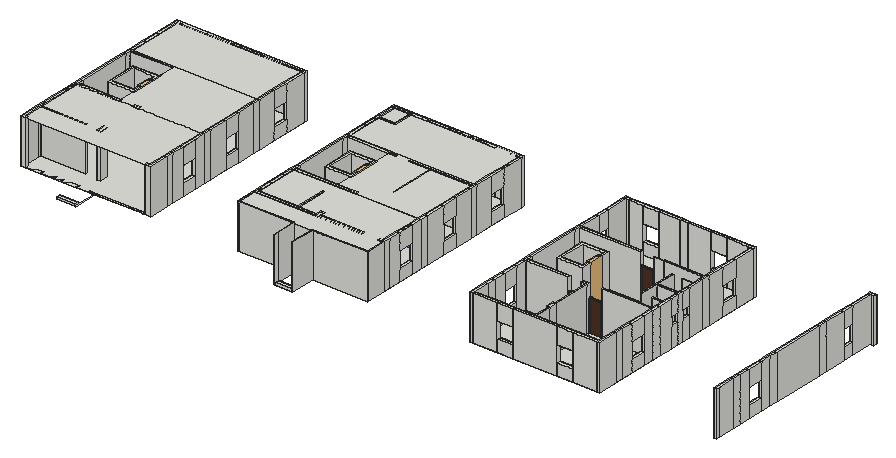
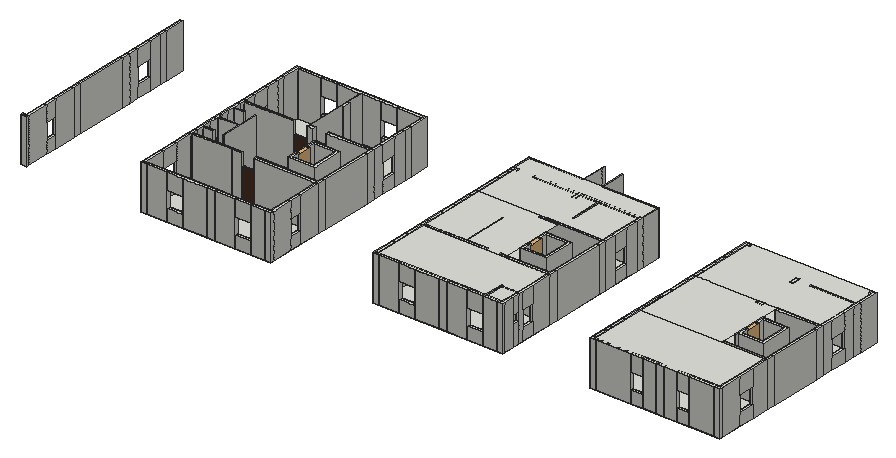
# SketchUp Ruby script. Lengths in inches.
U = 1.inch
M = Sketchup.active_model
def pt(a) = Geom::Point3d.new(a.map { |v| v * U })
def face(e, loops, mat)
  f = e.add_face(loops[0].map { |a| pt(a) })
  loops[1..].each { |l| e.add_face(l.map { |a| pt(a) }).erase! }
  f.material = f.back_material = mat if mat
  f
end
# faces: each face lists its corners as indices into pts; further lists are holes
def faces(e, pts, list, mat = nil) = list.each { |f| face(e, (f[0].is_a?(Array) ? f : [f]).map { |l| l.map { |i| pts[i] } }, mat) }
# xy, xz, yz: faces in a plane at the given z, y or x. An outline is a flat list of corners, or four numbers for a rectangle; further outlines are holes
def ring(l) = l.size == 4 ? [[l[0], l[1]], [l[2], l[1]], [l[2], l[3]], [l[0], l[3]]] : l.each_slice(2).to_a
def flat(e, list, mat, &to3) = list.each { |f| face(e, (f[0].is_a?(Array) ? f : [f]).map { |l| ring(l).map { |u, v| to3.(u, v) } }, mat) }
def xy(e, z, list, mat = nil) = flat(e, list, mat) { |x, y| [x, y, z] }
def xz(e, y, list, mat = nil) = flat(e, list, mat) { |x, z| [x, y, z] }
def yz(e, x, list, mat = nil) = flat(e, list, mat) { |y, z| [x, y, z] }
def lines(e, pts, list) = list.each { |a, b| e.add_line(pt(pts[a]), pt(pts[b])) }
# prism: a flat outline (further loops are holes) pulled along v
def prism(e, loops, v, mat = nil)
  f = face(e, loops, mat); d = Geom::Vector3d.new(v.map { |x| x * U })
  f.pushpull(f.normal.samedirection?(d) ? d.length : -d.length)
end
def box(e, o, s, mat = nil) = prism(e, [[o, [o[0] + s[0], o[1], o[2]], [o[0] + s[0], o[1] + s[1], o[2]], [o[0], o[1] + s[1], o[2]]]], [0, 0, s[2]], mat)
def at(x, y, z, deg = 0) = Geom::Transformation.translation(pt([x, y, z])) * Geom::Transformation.rotation(ORIGIN, Z_AXIS, deg.degrees)
def axes(o, x, y, z) = Geom::Transformation.new([*x, 0, *y, 0, *z, 0, *pt(o).to_a, 1])
def part(name) = M.definitions.add(name)
# library, detail: a bought-in or finely detailed component or shape, given as its bounding box
def library(name, o, s) = part(name).tap { |d| box(d.entities, o, s) }
def detail(e, o, s) = box(e.add_group.entities, o, s)
def put(e, d, t, mat = nil) = e.add_instance(d, t).tap { |i| i.material = mat if mat }
def group(e, t, mat = nil) = e.add_group.tap { |g| g.transformation = t; g.material = mat if mat }.entities
root = M.entities
M.materials.add("Polis06_194").color = [79, 50, 36]
M.materials.add("[Metal Aluminum Anodized]").color = [202, 209, 219]
M.materials.add("[Translucent Glass Blue]").color = [100, 149, 237]
M.materials["[Translucent Glass Blue]"].alpha = 0.5
c1 = library("lift",[-933.37,365.14,432],[57.92,12.32,108.27])
c2 = part("Group\#210")
box(c2.entities,[0,0,0],[12,46.92,6])
c3 = part("Group\#339")
box(c3.entities,[0,0,0],[55,12,6])
c4 = library("Flush door assembly",[0,0,0],[5.12,30.08,83.9375])
c5 = part("Flush door assembly \#1")
xy(c5.entities,0,[[0,0,4.72,1.18],[0,34.25,4.72,35.43]],"Polis06_194")
xy(c5.entities,85.26,[[0,1.18,4.72,34.25]],"Polis06_194")
xy(c5.entities,86.61,[[0,0,4.72,35.43]],"Polis06_194")
xz(c5.entities,0,[[0,0,4.72,86.61]],"Polis06_194")
xz(c5.entities,1.18,[[0,0,2.36,85.26],[2.36,0,4.72,85.26]],"Polis06_194")
xz(c5.entities,34.25,[[0,0,4.72,85.26]],"Polis06_194")
xz(c5.entities,35.43,[[0,0,4.72,86.61]],"Polis06_194")
yz(c5.entities,0,[[0,0,1.18,86.61],[34.25,0,35.43,86.61],[1.18,85.26,34.25,86.61]],"Polis06_194")
yz(c5.entities,2.36,[[1.18,0,34.25,0,34.25,85.21,1.18,85.26]],"Polis06_194")
yz(c5.entities,4.72,[[0,0,1.18,86.61],[34.25,0,35.43,86.61],[1.18,85.26,34.25,86.61]],"Polis06_194")
c6 = part("Group\#267")
box(c6.entities,[0,0,0],[52,12,6])
c7 = part("window")
xy(c7.entities,3.83,[[63.5,0,92.75,0.45],[92.75,0,122,0.23]],"[Metal Aluminum Anodized]")
xy(c7.entities,6,[[8,-0.1,32,0.24],[66,0,90.25,0.45],[95.25,0,119.5,0.23]],"[Metal Aluminum Anodized]")
xy(c7.entities,89.5,[[8,-0.1,32,0.24],[66,0,90.25,0.45],[95.25,0,119.5,0.23]],"[Metal Aluminum Anodized]")
xy(c7.entities,92,[[5.5,-0.1,34.5,0.24],[34.5,0,63.5,0.35],[63.5,0,92.75,0.45],[92.75,0,122,0.23]],"[Metal Aluminum Anodized]")
xz(c7.entities,-0.1,[[8,6,32,89.5]],"[Translucent Glass Blue]")
xz(c7.entities,0,[[63.5,3.5,92.75,3.83],[92.75,3.5,122,3.83]],"[Metal Aluminum Anodized]")
xz(c7.entities,0,[[66,6,90.25,89.5],[95.25,6,119.5,89.5]],"[Translucent Glass Blue]")
xz(c7.entities,0.23,[[[92.75,3.83,122,92],[95.25,6,119.5,89.5]]],"[Metal Aluminum Anodized]")
xz(c7.entities,0.24,[[[5.5,3.83,34.5,92],[8,6,32,89.5]]],"[Metal Aluminum Anodized]")
xz(c7.entities,0.45,[[[63.5,3.83,92.75,92],[66,6,90.25,89.5]]],"[Metal Aluminum Anodized]")
xz(c7.entities,0.45,[[[37,6,61,89.5],[39.25,48.08,39.64,48.15,40.01,48.35,40.32,48.67,40.5625,49.08,40.71,49.57,40.77,50.08,40.71,50.6,40.5625,51.08,40.32,51.5,40.01,51.82,39.64,52.02,39.25,52.08,38.86,52.02,38.49,51.82,38.18,51.5,37.94,51.08,37.79,50.6,37.74,50.08,37.79,49.57,37.94,49.08,38.18,48.67,38.49,48.35,38.86,48.15]]],"[Translucent Glass Blue]")
xz(c7.entities,0.8,[[[34.5,3.83,63.5,92],[37,6,61,89.5]]],"[Metal Aluminum Anodized]")
xz(c7.entities,2.08,[[39.25,48.08,38.86,48.15,38.49,48.35,38.18,48.67,37.94,49.08,37.79,49.57,37.74,50.08,37.79,50.6,37.94,51.08,38.18,51.5,38.49,51.82,38.86,52.02,39.25,52.08,39.64,52.02,40.01,51.82,40.32,51.5,40.5625,51.08,40.71,50.6,40.77,50.08,40.71,49.57,40.5625,49.08,40.32,48.67,40.01,48.35,39.64,48.15]],"[Metal Aluminum Anodized]")
yz(c7.entities,8,[[-0.1,6,0.24,89.5]],"[Metal Aluminum Anodized]")
yz(c7.entities,32,[[-0.1,6,0.24,89.5]],"[Metal Aluminum Anodized]")
yz(c7.entities,34.5,[[0.24,3.83,0.35,92]],"[Metal Aluminum Anodized]")
yz(c7.entities,61,[[0.45,6,0.8,89.5]],"[Metal Aluminum Anodized]")
yz(c7.entities,63.5,[[0.35,3.83,0.45,92]],"[Metal Aluminum Anodized]")
yz(c7.entities,66,[[0,6,0.45,89.5]],"[Metal Aluminum Anodized]")
yz(c7.entities,90.25,[[0,6,0.45,89.5]],"[Metal Aluminum Anodized]")
yz(c7.entities,92.75,[[0.23,3.83,0.45,92]],"[Metal Aluminum Anodized]")
yz(c7.entities,95.25,[[0,6,0.23,89.5]],"[Metal Aluminum Anodized]")
yz(c7.entities,119.5,[[0,6,0.23,89.5]],"[Metal Aluminum Anodized]")
yz(c7.entities,122,[[0,3.83,0.23,92]],"[Metal Aluminum Anodized]")
p = [[39.25,0.45,48.08],[38.86,0.45,48.15],[38.86,2.08,48.15],[39.25,2.08,48.08],[39.64,0.45,48.15],[39.64,2.08,48.15],
  [38.49,0.45,48.35],[38.49,2.08,48.35],[40.01,0.45,48.35],[40.01,2.08,48.35],[38.18,0.45,48.67],[38.18,2.08,48.67],
  [40.32,0.45,48.67],[40.32,2.08,48.67],[37.94,0.45,49.08],[37.94,2.08,49.08],[40.5625,0.45,49.08],[40.5625,2.08,49.08],
  [37.79,0.45,49.57],[37.79,2.08,49.57],[40.71,0.45,49.57],[40.71,2.08,49.57],[37.74,0.45,50.08],[37.74,2.08,50.08],
  [40.77,0.45,50.08],[40.77,2.08,50.08],[37.79,0.45,50.6],[37.79,2.08,50.6],[40.71,0.45,50.6],[40.71,2.08,50.6],
  [37.94,0.45,51.08],[37.94,2.08,51.08],[40.5625,0.45,51.08],[40.5625,2.08,51.08],[38.18,0.45,51.5],[38.18,2.08,51.5],
  [40.32,0.45,51.5],[40.32,2.08,51.5],[38.49,0.45,51.82],[38.49,2.08,51.82],[40.01,0.45,51.82],[40.01,2.08,51.82],
  [38.86,0.45,52.02],[38.86,2.08,52.02],[39.64,0.45,52.02],[39.64,2.08,52.02],[39.25,0.45,52.08],[39.25,2.08,52.08],
  [94.5,0,6],[95.25,0,6],[125.5,0,3.5],[125.5,0,3.83],[125.5,10,3.5],[125.5,10,3.83],
  [34.5,0.35,3.83],[63.5,0.35,3.83],[32,-0.1,6],[33.75,-0.1,6],[34.5,-0.1,3.83],[34.5,0.24,3.83],
  [63.5,0.9,3.83],[63.5,0.9,92]]
faces(c7.entities,p,[[0,1,2,3],[4,0,3,5],[1,6,7,2],[8,4,5,9],[6,10,11,7],[12,8,9,13],[10,14,15,11],[16,12,13,17],
  [14,18,19,15],[20,16,17,21],[18,22,23,19],[24,20,21,25],[22,26,27,23],[28,24,25,29],[26,30,31,27],[32,28,29,33],
  [30,34,35,31],[36,32,33,37],[34,38,39,35],[40,36,37,41],[38,42,43,39],[44,40,41,45],[42,46,47,43],[46,44,45,47]],"[Metal Aluminum Anodized]")
lines(c7.entities,p,[[48,49],[50,51],[52,53],[54,55],[56,57],[58,59],[60,61]])
xy(root,0,[[809.93,0,812.93,72],[864.93,0,867.93,72],[200.53,72,219.62,73],[219.62,72,222.62,73],[222.62,72,369.69,73],
  [645.31,72,809.93,75],[812.93,72,864.93,72,864.93,75,1029.55,75,1029.55,131.04,1032.55,131.04,1032.55,652.56,645.31,652.56,645.31,131.04,648.31,131.04,648.31,75,812.93,75],[809.93,72,812.93,75],[864.93,72,867.93,75],[867.93,72,1032.55,75],
  [1334.55,72,1721.79,652.56],[[0,73,200.53,73,200.53,81,369.69,81,369.69,73,386.24,73,386.24,652.56,0,652.56],[9,137.04,142.44,140.04]],[200.53,73,219.62,73,219.62,75,222.62,75,222.62,73,369.69,73,369.69,81,200.53,81],[219.62,73,222.62,75],[645.31,75,648.31,131.04],
  [1029.55,75,1032.55,131.04],[9,137.04,142.44,140.04]])
xy(root,132,[[809.93,0,812.93,72],[864.93,0,867.93,72],[[0,72,387.24,270],[9,137.04,142.44,140.04]],[645.31,72,809.93,75],[[809.93,72,867.93,72,867.93,75,1029.55,75,1029.55,131.04,1032.55,131.04,1032.55,270,645.31,270,645.31,131.04,648.31,131.04,648.31,75,809.93,75],[654.31,137.04,787.75,140.04]],
  [867.93,72,1032.55,75],[645.31,75,648.31,131.04],[1029.55,75,1032.55,131.04],[9,137.04,142.44,140.04],[135,270,378.24,477.12],
  [780.31,270,1023.55,477.12],[0,477.12,387.24,652.56],[645.31,477.12,1032.55,652.56]])
xz(root,0,[[809.93,0,812.93,132],[864.93,0,867.93,132]])
xz(root,72,[[645.31,0,809.93,132],[809.93,0,812.93,132],[864.93,0,867.93,132],[867.93,0,1032.55,132]])
xz(root,75,[[645.31,0,648.31,132],[648.31,0,797.93,132],[797.93,0,809.93,132],[867.93,0,879.93,132],[879.93,0,1029.55,132],
  [1029.55,0,1032.55,132]])
xz(root,131.04,[[645.31,0,648.31,132],[1029.55,0,1032.55,132]])
xz(root,137.04,[[9,0,142.44,132]])
xz(root,140.04,[[9,0,142.44,132]])
yz(root,9,[[137.04,0,140.04,132]])
yz(root,142.44,[[137.04,0,140.04,132]])
yz(root,645.31,[[72,0,75,132],[75,0,131.04,132]])
yz(root,648.31,[[75,0,131.04,132]])
yz(root,809.93,[[0,0,72,132],[72,0,75,132]])
yz(root,812.93,[[0,0,12,132],[12,0,72,132]])
yz(root,864.93,[[0,0,12,132],[12,0,72,132]])
yz(root,867.93,[[0,0,72,132],[72,0,75,132]])
yz(root,1029.55,[[75,0,131.04,132]])
yz(root,1032.55,[[72,0,75,132],[75,0,131.04,132]])
g1 = group(root,at(0,190.68,0))
box(g1,[0,0,0],[9,47.4,36])
box(g1,[0,0,84],[9,47.4,48])
p = [[9,0,36],[9,0,84],[9,47.4,36],[9,47.4,84]]
lines(g1,p,[[0,1],[2,3]])
g2 = group(root,at(0,530.64,0))
box(g2,[0,0,0],[9,47.16,36])
box(g2,[0,0,84],[9,47.16,48])
p = [[9,0,36],[9,0,84],[9,47.16,36],[9,47.16,84]]
lines(g2,p,[[0,1],[2,3]])
g3 = group(root,at(0,477.12,0))
box(g3,[0,0,0],[9,53.52,132])
g4 = group(root,at(0,577.8,0))
box(g4,[0,0,0],[9,65.76,132])
g5 = group(root,at(0,270,0))
prism(g5,[[[9,0,0],[0,0,0],[0,24,0],[9,24,0],[9,9,0]]],[0,0,132])
g6 = group(root,at(0,238.08,0))
box(g6,[0,0,0],[9,31.92,132])
g7 = group(root,at(0,131.04,0))
prism(g7,[[[0,0,0],[0,24,0],[9,24,0],[9,9,0],[9,6,0],[9,0,0]]],[0,0,132])
g8 = group(root,at(0,453.12,0))
prism(g8,[[[9,0,0],[0,0,0],[0,24,0],[9,24,0],[9,18,0],[9,15,0]]],[0,0,132])
g9 = group(root,at(0,155.04,0))
box(g9,[0,0,0],[9,35.64,132])
g10 = group(root,at(0,294,0))
box(g10,[0,0,0],[9,159.12,132])
g11 = group(root,at(0,72,0))
prism(g11,[[[16.12,0,0],[0,0,0],[0,59.04,0],[9,59.04,0],[9,9,0],[16.12,9,0]]],[0,0,132])
g12 = group(root,at(0,643.56,0))
box(g12,[0,0,0],[18,9,132])
g13 = group(root,at(18,643.56,0))
box(g13,[0,0,0],[76.2,9,132])
g14 = group(root,at(9,270,0))
box(g14,[0,0,0],[126,9,132])
g15 = group(root,at(9,468.12,0))
box(g15,[0,0,0],[126,3,132])
g16 = group(root,at(9,140.04,0))
p = [[0,0,0],[133.44,0,0]]
lines(g16,p,[[0,1]])
g17 = group(root,at(16.12,72,0))
xy(g17,0,[[0,0,152.6,9]])
g18 = group(root,at(55.92,325.92,0))
prism(g18,[[[79.08,95.28,0],[79.08,65.64,0],[70.08,65.64,0],[70.08,86.28,0],[9,86.28,0],[9,9,0],[70.08,9,0],[70.08,29.64,0],[79.08,29.64,0],[79.08,0,0],[0,0,0],[0,95.28,0]]],[0,0,132])
g19 = group(root,at(94.2,643.56,0))
box(g19,[0,0,0],[35.64,9,36])
box(g19,[0,0,84],[35.64,9,48])
p = [[0,0,36],[0,0,84],[35.64,0,36],[35.64,0,84]]
lines(g19,p,[[0,1],[2,3]])
put(root,c1,axes([500.14,1008.92,-527.04],[0,0.7,0],[-1,0,0],[0,0,1.22]))
put(root,c2,at(123,279,0))
g20 = group(root,at(132,421.2,0))
box(g20,[0,0,0],[3,7.92,132])
g21 = group(root,at(129.84,643.56,0))
box(g21,[0,0,0],[38.04,9,132])
g22 = group(root,at(167.88,643.56,0))
box(g22,[0,0,0],[24,9,132])
g23 = group(root,at(173.88,270,0))
box(g23,[0,0,0],[18,9,132])
g24 = group(root,at(168.71,72,0))
xy(g24,0,[[0,0,31.82,9]])
g25 = group(root,at(181.44,131.04,0))
box(g25,[0,0,0],[10.44,24,132])
put(root,c3,at(164.62,0,0))
g26 = group(root,at(191.88,643.56,0))
box(g26,[0,0,0],[38.04,9,132])
g27 = group(root,at(219.62,0,0))
xy(g27,0,[[0,0,3,72]])
g28 = group(root,at(229.92,643.56,0))
box(g28,[0,0,0],[35.4,9,36])
box(g28,[0,0,84],[35.4,9,48])
p = [[0,0,36],[0,0,84],[35.4,0,36],[35.4,0,84]]
lines(g28,p,[[0,1],[2,3]])
g29 = group(root,at(265.32,643.56,0))
box(g29,[0,0,0],[103.92,9,132])
g30 = group(root,at(369.24,643.56,0))
box(g30,[0,0,0],[18,9,132])
g31 = group(root,at(369.69,72,0))
prism(g31,[[[8.55,9,0],[8.55,59.04,0],[17.55,59.04,0],[17.55,0,0],[0,0,0],[0,9,0]]],[0,0,132])
g32 = group(root,at(378.24,577.8,0))
box(g32,[0,0,0],[9,65.76,132])
g33 = group(root,at(378.24,294,0))
box(g33,[0,0,0],[9,58.92,132])
g34 = group(root,at(378.24,238.08,0))
box(g34,[0,0,0],[9,31.92,132])
g35 = group(root,at(378.24,190.68,0))
box(g35,[0,0,0],[9,47.4,36])
box(g35,[0,0,84],[9,47.4,48])
p = [[0,47.4,36],[0,47.4,84],[0,0,36],[0,0,84]]
lines(g35,p,[[0,1],[2,3]])
g36 = group(root,at(378.24,155.04,0))
box(g36,[0,0,0],[9,35.64,132])
g37 = group(root,at(378.24,352.92,0))
box(g37,[0,0,0],[9,47.4,36])
box(g37,[0,0,84],[9,47.4,48])
p = [[0,47.4,36],[0,47.4,84],[0,0,36],[0,0,84]]
lines(g37,p,[[0,1],[2,3]])
g38 = group(root,at(378.24,530.64,0))
box(g38,[0,0,0],[9,47.16,36])
box(g38,[0,0,84],[9,47.16,48])
p = [[0,47.16,36],[0,47.16,84],[0,0,36],[0,0,84]]
lines(g38,p,[[0,1],[2,3]])
g39 = group(root,at(378.24,131.04,0))
box(g39,[0,0,0],[9,24,132])
g40 = group(root,at(378.24,270,0))
box(g40,[0,0,0],[9,24,132])
g41 = group(root,at(378.24,453.12,0))
box(g41,[0,0,0],[9,24,132])
g42 = group(root,at(378.24,477.12,0))
box(g42,[0,0,0],[9,53.52,132])
g43 = group(root,at(378.24,400.32,0))
box(g43,[0,0,0],[9,52.8,132])
g44 = group(root,at(645.31,541.84,0))
box(g44,[0,0,0],[9,35.96,36])
box(g44,[0,0,84],[9,35.96,48])
p = [[9,35.96,36],[9,35.96,84],[9,0,36],[9,0,84]]
lines(g44,p,[[0,1],[2,3]])
g45 = group(root,at(645.31,477.12,0))
box(g45,[0,0,0],[9,64.72,132])
g46 = group(root,at(645.31,270,0))
box(g46,[0,0,0],[9,24,132])
g47 = group(root,at(645.31,294,0))
box(g47,[0,0,0],[9,159.12,132])
g48 = group(root,at(645.31,155.04,0))
xy(g48,0,[[0,0,9,35.64],[0,35.64,9,83.04],[0,83.04,9,114.96]])
xy(g48,36,[[0,35.64,9,83.04]])
xy(g48,84,[[0,35.64,9,83.04]])
xy(g48,132,[[0,0,9,35.64],[0,35.64,9,83.04],[0,83.04,9,114.96]])
xz(g48,0,[[0,0,9,132]])
xz(g48,35.64,[[0,0,9,36],[0,36,9,84],[0,84,9,132]])
xz(g48,83.04,[[0,0,9,36],[0,36,9,84],[0,84,9,132]])
xz(g48,114.96,[[0,0,9,132]])
yz(g48,0,[[0,0,35.64,132],[35.64,0,83.04,36],[83.04,0,114.96,132],[35.64,84,83.04,132]])
yz(g48,9,[[0,0,35.64,132],[35.64,0,83.04,36],[83.04,0,114.96,132],[35.64,84,83.04,132]])
g49 = group(root,at(645.31,131.04,0))
box(g49,[0,0,0],[9,24,132])
g50 = group(root,at(645.31,453.12,0))
box(g50,[0,0,0],[9,24,132])
g51 = group(root,at(645.31,617.34,0))
box(g51,[0,0,0],[9,26.22,132])
g52 = group(root,at(645.31,593.38,0))
box(g52,[0,0,0],[9,23.96,60])
box(g52,[0,0,84],[9,23.96,48])
p = [[9,23.96,60],[9,23.96,84],[9,0,60],[9,0,84]]
lines(g52,p,[[0,1],[2,3]])
g53 = group(root,at(645.31,577.8,0))
box(g53,[0,0,0],[9,15.58,132])
g54 = group(root,at(645.31,643.56,0))
box(g54,[0,0,0],[18,9,132])
g55 = group(root,at(654.31,584.34,0))
box(g55,[0,0,0],[15.3,4.5,132])
g56 = group(root,at(663.31,584.34,0))
prism(g56,[[[40.8,68.22,0],[40.8,0,0],[36.3,0,0],[36.3,59.22,0],[0,59.22,0],[0,68.22,0]]],[0,0,132])
put(root,c4,at(699.61,583.72,0,90))
g57 = group(root,at(669.61,584.34,0))
box(g57,[0,0,84],[30,4.5,48])
box(g57,[0,0,-0.04],[30,4.5,0.04])
p = [[30,4.5,84],[30,4.5,0],[0,4.5,84],[0,4.5,0]]
lines(g57,p,[[0,1],[2,3]])
g58 = group(root,at(654.31,468.12,0))
prism(g58,[[[118.92,0,0],[0,0,0],[0,9,0],[118.92,9,0],[118.92,3,0]]],[0,0,132])
g59 = group(root,at(704.11,643.56,0))
box(g59,[0,0,0],[47.64,9,36])
box(g59,[0,0,84],[47.64,9,48])
p = [[47.64,0,36],[47.64,0,84],[0,0,36],[0,0,84]]
lines(g59,p,[[0,1],[2,3]])
g60 = group(root,at(654.31,270,0))
box(g60,[0,0,0],[164.88,9,132])
g61 = group(root,at(654.31,131.04,0))
prism(g61,[[[0,9,0],[116,9,0],[120,9,0],[172.44,9,0],[172.44,0,0],[0,0,0]]],[0,0,132])
g62 = group(root,at(701.23,325.92,0))
prism(g62,[[[9,9,0],[70.08,9,0],[70.08,29.64,0],[79.08,29.64,0],[79.08,0,0],[0,0,0],[0,95.28,0],[79.08,95.28,0],[79.08,65.64,0],[70.08,65.64,0],[70.08,86.28,0],[9,86.28,0]]],[0,0,132])
put(root,c5,axes([774.31,270,0],[-1,0,0],[0,-1.10067,0],[0,0,1.10836]))
g63 = group(root,at(770.31,140.04,0))
box(g63,[0,0,0],[4,91.125,132])
put(root,c1,axes([1145.45,1008.92,-527.04],[0,0.7,0],[-1,0,0],[0,0,1.22]))
put(root,c2,at(768.31,279,0))
g64 = group(root,at(751.75,643.56,0))
box(g64,[0,0,0],[61.44,9,132])
g65 = group(root,at(773.23,468.12,0))
box(g65,[0,0,0],[24.96,3,132])
put(root,c5,axes([837.19,468.12,0],[0,1,0],[-1.10067,0,0],[0,0,1.10836]))
g66 = group(root,at(813.19,643.56,0))
box(g66,[0,0,0],[24,9,132])
g67 = group(root,at(819.19,270,0))
box(g67,[0,0,0],[18,9,132])
g68 = group(root,at(826.75,131.04,0))
box(g68,[0,0,0],[10.44,24,132])
put(root,c6,at(812.93,0,0))
g69 = group(root,at(837.19,643.56,0))
box(g69,[0,0,0],[69,9,132])
g70 = group(root,at(837.19,131.04,0))
box(g70,[0,0,0],[129.36,9,132])
put(root,c7,axes([900.55,473.99,-5.22],[0,-1.15951,0],[1,0,0],[0,0,1.49]))
g71 = group(root,at(906.19,643.56,0))
box(g71,[0,0,0],[47.4,9,36])
box(g71,[0,0,84],[47.4,9,48])
p = [[0,0,36],[0,0,84],[47.4,0,36],[47.4,0,84]]
lines(g71,p,[[0,1],[2,3]])
g72 = group(root,at(837.19,468.12,0))
box(g72,[0,0,0],[186.36,3,132])
put(root,c7,axes([895.96,331.92,-8.94],[1.0541,0,0],[0,1,0],[0,0,1.49]))
g73 = group(root,at(953.59,643.56,0))
box(g73,[0,0,0],[60.96,9,132])
put(root,c5,axes([1014.55,131.04,0],[0,1,0],[-1.35467,0,0],[0,0,1.10836]))
g74 = group(root,at(1014.55,131.04,0))
box(g74,[0,0,0],[9,9,132])
g75 = group(root,at(1014.55,643.56,0))
box(g75,[0,0,0],[18,9,132])
g76 = group(root,at(1023.55,530.64,0))
box(g76,[0,0,0],[9,47.16,36])
box(g76,[0,0,84],[9,47.16,48])
p = [[0,47.16,36],[0,47.16,84],[0,0,36],[0,0,84]]
lines(g76,p,[[0,1],[2,3]])
g77 = group(root,at(1023.55,577.8,0))
box(g77,[0,0,0],[9,65.76,132])
g78 = group(root,at(1023.55,400.32,0))
box(g78,[0,0,0],[9,52.8,132])
g79 = group(root,at(1023.55,294,0))
box(g79,[0,0,0],[9,58.92,132])
g80 = group(root,at(1023.55,238.08,0))
box(g80,[0,0,0],[9,31.92,132])
g81 = group(root,at(1023.55,155.04,0))
box(g81,[0,0,0],[9,35.64,132])
g82 = group(root,at(1023.55,477.12,0))
box(g82,[0,0,0],[9,53.52,132])
g83 = group(root,at(1023.55,352.92,0))
box(g83,[0,0,0],[9,47.4,36])
box(g83,[0,0,84],[9,47.4,48])
p = [[0,47.4,36],[0,47.4,84],[0,0,36],[0,0,84]]
lines(g83,p,[[0,1],[2,3]])
g84 = group(root,at(1023.55,131.04,0))
box(g84,[0,0,0],[9,24,132])
g85 = group(root,at(1023.55,270,0))
box(g85,[0,0,0],[9,24,132])
g86 = group(root,at(1023.55,453.12,0))
box(g86,[0,0,0],[9,24,132])
g87 = group(root,at(1023.55,190.68,0))
box(g87,[0,0,0],[9,47.4,36])
box(g87,[0,0,84],[9,47.4,48])
p = [[0,0,36],[0,0,84],[0,47.4,36],[0,47.4,84]]
lines(g87,p,[[0,1],[2,3]])
g88 = group(root,at(1334.55,238.08,0))
box(g88,[0,0,-0.33],[9,31.92,132.33])
g89 = group(root,at(1334.55,577.8,0))
box(g89,[0,0,0],[9,65.76,132])
g90 = group(root,at(1334.55,541.88,0))
box(g90,[0,0,0],[9,35.92,36])
box(g90,[0,0,84],[9,35.92,48])
p = [[9,0,36],[9,0,84],[9,35.92,36],[9,35.92,84]]
lines(g90,p,[[0,1],[2,3]])
g91 = group(root,at(1334.55,270,0))
box(g91,[0,0,0],[9,24,132])
g92 = group(root,at(1334.55,294,0))
box(g92,[0,0,0],[9,159.12,132])
g93 = group(root,at(1334.55,155.04,0))
box(g93,[0,0,0],[9,35.64,132])
g94 = group(root,at(1334.55,72,0))
prism(g94,[[[9,59.04,0],[9,9,0],[9,0,0],[0,0,0],[0,59.04,0]]],[0,0,132])
g95 = group(root,at(1334.55,477.12,0))
box(g95,[0,0,0],[9,64.76,132])
g96 = group(root,at(1334.55,190.68,0))
box(g96,[0,0,0],[9,47.4,36])
box(g96,[0,0,84],[9,47.4,48])
p = [[9,47.4,36],[9,47.4,84],[9,0,36],[9,0,84]]
lines(g96,p,[[0,1],[2,3]])
g97 = group(root,at(1334.55,453.12,0))
box(g97,[0,0,0],[9,24,132])
g98 = group(root,at(1334.55,131.04,0))
box(g98,[0,0,0],[9,24,132])
g99 = group(root,at(1334.55,643.56,0))
box(g99,[0,0,0],[18,9,132])
g100 = group(root,at(1352.55,643.56,0))
box(g100,[0,0,0],[40.8,9,132])
g101 = group(root,at(1343.55,72,0))
box(g101,[0,0,0],[73.2,9,132])
g102 = group(root,at(1343.55,270,0))
box(g102,[0,0,0],[126,9,132])
g103 = group(root,at(1393.35,643.56,0))
box(g103,[0,0,0],[47.64,9,36])
box(g103,[0,0,84],[47.64,9,48])
p = [[0,0,36],[0,0,84],[47.64,0,36],[47.64,0,84]]
lines(g103,p,[[0,1],[2,3]])
g104 = group(root,at(1390.47,325.92,0))
prism(g104,[[[0,95.28,0],[79.08,95.28,0],[79.08,65.64,0],[70.08,65.64,0],[70.08,86.28,0],[9,86.28,0],[9,9,0],[70.08,9,0],[70.08,29.64,0],[79.08,29.64,0],[79.08,0,0],[0,0,0]]],[0,0,132])
g105 = group(root,at(1343.55,468.12,0))
box(g105,[0,0,0],[182.88,9,132])
g106 = group(root,at(1416.75,72,0))
box(g106,[0,0,0],[47.64,9,36])
box(g106,[0,0,84],[47.64,9,48])
p = [[0,9,36],[0,9,84],[47.64,9,36],[47.64,9,84]]
lines(g106,p,[[0,1],[2,3]])
put(root,c1,axes([1834.69,1008.92,-527.04],[0,0.7,0],[-1,0,0],[0,0,1.22]))
put(root,c2,at(1457.55,279,0))
g107 = group(root,at(1440.99,643.56,0))
box(g107,[0,0,0],[61.44,9,132])
put(root,c5,axes([1508.43,270,0],[0,1,0],[-1.10067,0,0],[0,0,1.10836]))
g108 = group(root,at(1502.43,643.56,0))
box(g108,[0,0,0],[24,9,132])
g109 = group(root,at(1508.43,270,0))
box(g109,[0,0,0],[18,9,132])
g110 = group(root,at(1515.99,131.04,0))
box(g110,[0,0,0],[10.44,24,132])
g111 = group(root,at(1522.43,81,0))
box(g111,[0,0,0],[4,50.04,132])
g112 = group(root,at(1522.43,155.04,0))
box(g112,[0,0,0],[4,114.96,132])
g113 = group(root,at(1464.39,72,0))
prism(g113,[[[62.04,9,0],[131.04,9,0],[131.04,0,0],[0,0,0],[0,9,0],[58.04,9,0]]],[0,0,132])
put(root,c5,axes([1565.43,468.12,0],[0,1,0],[-1.10067,0,0],[0,0,1.10836]))
put(root,c5,axes([1565.43,275,0],[0,1,0],[-1.10067,0,0],[0,0,1.10836]))
g114 = group(root,at(1526.43,643.56,0))
box(g114,[0,0,0],[69,9,132])
g115 = group(root,at(1565.43,468.12,0))
box(g115,[0,0,0],[29.36,3,132])
g116 = group(root,at(1595.43,72,0))
box(g116,[0,0,0],[47.4,9,36])
box(g116,[0,0,84],[47.4,9,48])
p = [[0,9,36],[0,9,84],[47.4,9,36],[47.4,9,84]]
lines(g116,p,[[0,1],[2,3]])
g117 = group(root,at(1595.43,643.56,0))
box(g117,[0,0,0],[47.4,9,36])
box(g117,[0,0,84],[47.4,9,48])
p = [[0,0,36],[0,0,84],[47.4,0,36],[47.4,0,84]]
lines(g117,p,[[0,1],[2,3]])
g118 = group(root,at(1565.43,275,0))
box(g118,[0,0,0],[147.36,4,132])
g119 = group(root,at(1648.29,315,0))
prism(g119,[[[4.5,56.31,0],[4.5,0,0],[0,0,0],[0,117.12,0],[4.5,117.12,0],[4.5,60.81,0]]],[0,0,132])
g120 = group(root,at(1594.79,468.12,0))
prism(g120,[[[0,3,0],[0,4.5,0],[118,4.5,0],[118,0,0],[0,0,0]]],[0,0,132])
put(root,c4,at(1682.79,430.45,0,90))
put(root,c4,at(1682.79,317.83,0,90))
g121 = group(root,at(1642.83,643.56,0))
box(g121,[0,0,0],[60.96,9,132])
g122 = group(root,at(1642.83,72,0))
box(g122,[0,0,0],[69.96,9,132])
g123 = group(root,at(1652.79,371.31,0))
box(g123,[0,0,0],[60,4.5,132])
g124 = group(root,at(1682.79,427.62,0))
box(g124,[0,0,0],[30,4.5,132])
g125 = group(root,at(1682.79,315,0))
box(g125,[0,0,0],[30,4.5,132])
g126 = group(root,at(1703.79,643.56,0))
box(g126,[0,0,0],[18,9,132])
g127 = group(root,at(1712.79,72,0))
prism(g127,[[[0,0,0],[0,9,0],[0,59.04,0],[9,59.04,0],[9,0,0]]],[0,0,132])
g128 = group(root,at(1712.79,339.05,0))
box(g128,[0,0,0],[9,24,60])
box(g128,[0,0,84],[9,24,48])
p = [[0,24,60],[0,24,84],[0,0,60],[0,0,84]]
lines(g128,p,[[0,1],[2,3]])
g129 = group(root,at(1712.79,477.12,0))
box(g129,[0,0,0],[9,53.52,132])
g130 = group(root,at(1712.79,530.64,0))
box(g130,[0,0,0],[9,47.16,36])
box(g130,[0,0,84],[9,47.16,48])
p = [[0,47.16,36],[0,47.16,84],[0,0,36],[0,0,84]]
lines(g130,p,[[0,1],[2,3]])
g131 = group(root,at(1712.79,577.8,0))
box(g131,[0,0,0],[9,65.76,132])
g132 = group(root,at(1712.79,190.68,0))
box(g132,[0,0,0],[9,47.4,36])
box(g132,[0,0,84],[9,47.4,48])
g133 = group(root,at(1712.79,238.08,0))
box(g133,[0,0,0],[9,31.92,132])
g134 = group(root,at(1712.79,294,0))
prism(g134,[[[0,45.05,0],[9,45.05,0],[9,0,0],[0,0,0],[0,21,0],[0,25.5,0]]],[0,0,132])
g135 = group(root,at(1712.79,405.66,0))
prism(g135,[[[9,47.46,0],[9,0,0],[0,0,0],[0,21.96,0],[0,26.46,0],[0,47.46,0]]],[0,0,132])
g136 = group(root,at(1712.79,453.12,0))
box(g136,[0,0,0],[9,24,132])
g137 = group(root,at(1712.79,270,0))
box(g137,[0,0,0],[9,24,132])
g138 = group(root,at(1712.79,131.04,0))
box(g138,[0,0,0],[9,24,132])
g139 = group(root,at(1712.79,155.04,0))
box(g139,[0,0,0],[9,35.64,132])
g140 = group(root,at(1712.79,381.7,0))
box(g140,[0,0,0],[9,23.96,60])
box(g140,[0,0,84],[9,23.96,48])
p = [[0,23.96,60],[0,23.96,84],[0,0,60],[0,0,84]]
lines(g140,p,[[0,1],[2,3]])
g141 = group(root,at(1712.79,363.05,0))
prism(g141,[[[0,18.65,0],[9,18.65,0],[9,0,0],[0,0,0],[0,8.26,0],[0,12.76,0]]],[0,0,132])
g142 = group(root,at(2061.45,577.8,0))
box(g142,[0,0,0],[9,65.76,132])
g143 = group(root,at(2061.45,477.12,0))
box(g143,[0,0,0],[9,64.76,132])
g144 = group(root,at(2061.45,541.88,0))
box(g144,[0,0,0],[9,35.92,36])
box(g144,[0,0,84],[9,35.92,48])
p = [[9,35.92,36],[9,35.92,84],[9,0,36],[9,0,84]]
lines(g144,p,[[0,1],[2,3]])
g145 = group(root,at(2061.45,453.12,0))
box(g145,[0,0,0],[9,24,132])
g146 = group(root,at(2061.45,238.08,0))
box(g146,[0,0,0],[9,31.92,132])
g147 = group(root,at(2061.45,155.04,0))
box(g147,[0,0,0],[9,35.64,132])
g148 = group(root,at(2061.45,72,0))
prism(g148,[[[0,0,0],[0,59.04,0],[9,59.04,0],[9,9,0],[9,0,0]]],[0,0,132])
g149 = group(root,at(2061.45,190.68,0))
box(g149,[0,0,0],[9,47.4,36])
box(g149,[0,0,84],[9,47.4,48])
p = [[9,47.4,36],[9,47.4,84],[9,0,36],[9,0,84]]
lines(g149,p,[[0,1],[2,3]])
g150 = group(root,at(2061.45,131.04,0))
box(g150,[0,0,0],[9,24,132])
g151 = group(root,at(2061.45,270,0))
box(g151,[0,0,0],[9,24,132])
g152 = group(root,at(2061.45,294,0))
box(g152,[0,0,0],[9,159.12,132])
g153 = group(root,at(2061.45,643.56,0))
box(g153,[0,0,0],[18,9,132])
